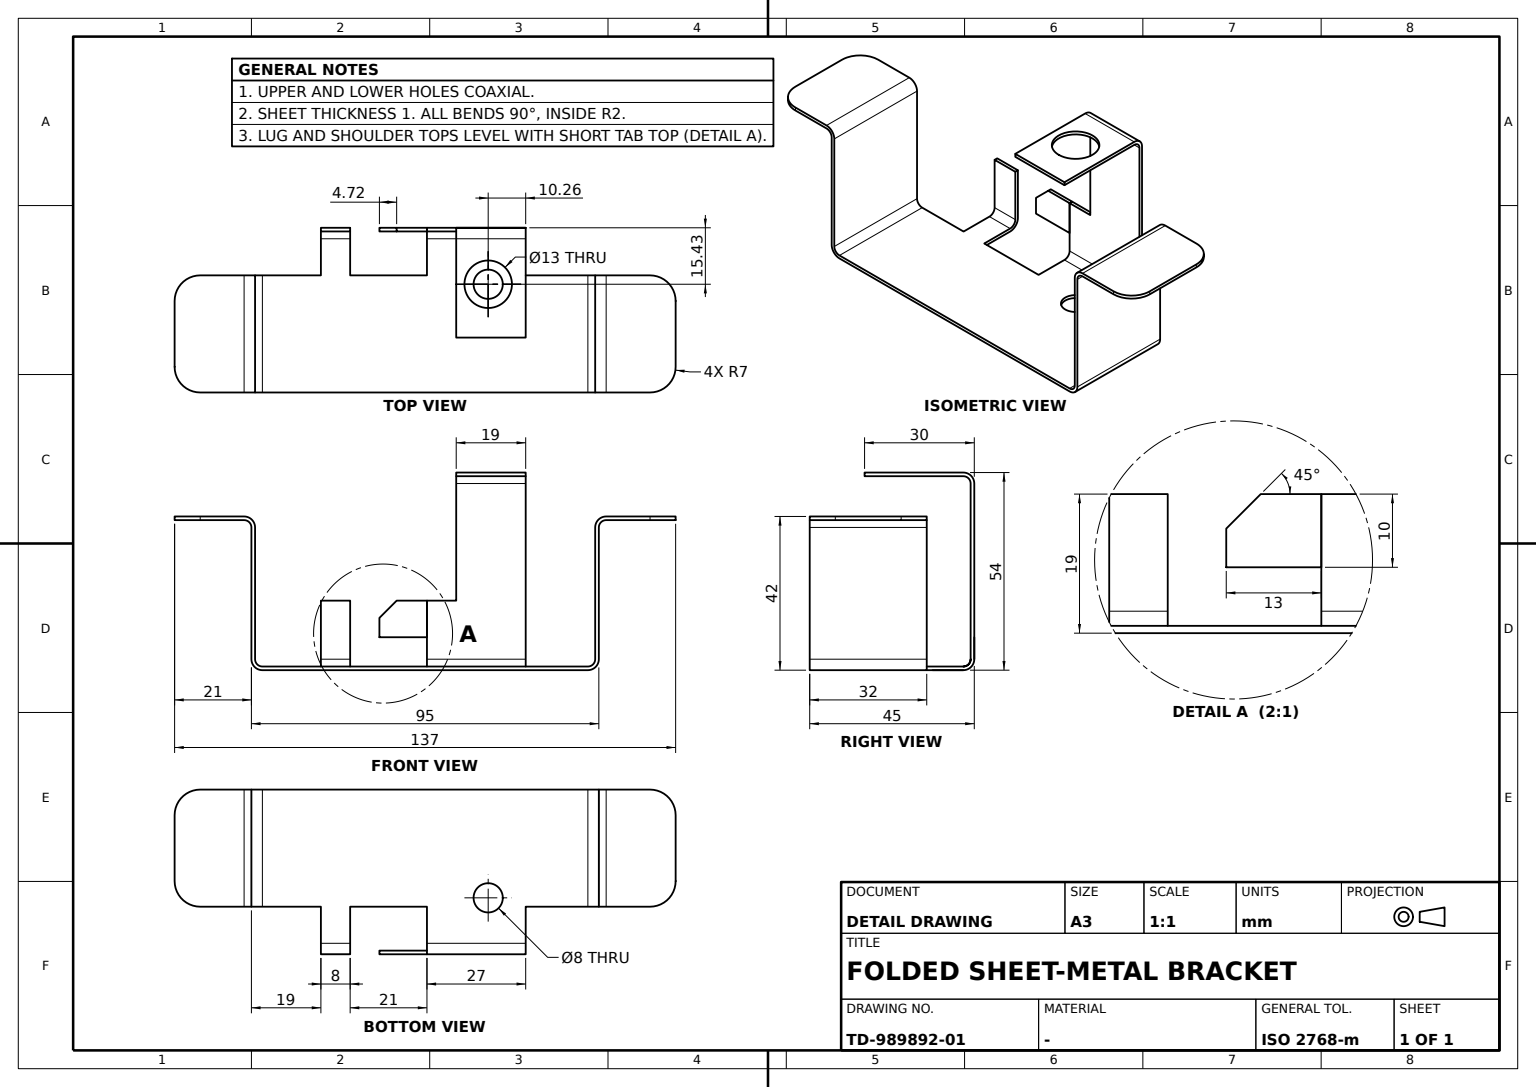
solid
v1 (27.5,26,53)
v2 (8.5,26,53)
e1 v1 v2 LINE
v3 (27.5,29,50)
e2 v3 v1 CIRCLE(AX(P(27.5,26,50),D(1,0,0),D(0,0,-1)),3)
v4 (8.5,29,50)
e3 v3 v4 LINE
e4 v4 v2 CIRCLE(AX(P(8.5,26,50),D(1,0,0),D(0,0,-1)),3)
face CYL(AX(P(18,26,50),D(-1,0,0),D(0,1,0)),3) [-e1 -e2 e3 e4]
v5 (-61.5,16,41)
v6 (-49.5,16,41)
e5 v5 v6 LINE
v7 (-68.5,9,41)
e6 v5 v7 CIRCLE(AX(P(-61.5,9,41),D(0,0,1),D(1,0,0)),7)
v8 (-68.5,-9,41)
e7 v8 v7 LINE
v9 (-61.5,-16,41)
e8 v8 v9 CIRCLE(AX(P(-61.5,-9,41),D(0,0,1),D(1,0,0)),7)
v10 (-49.5,-16,41)
e9 v10 v9 LINE
e10 v10 v6 LINE
face PLANE(AX(P(-47.5,0,41),D(0,0,1),D(0,1,0))) [-e5 e6 -e7 e8 -e9 e10]
v11 (-46.5,16,2)
v12 (-44.5,16,0)
e11 v11 v12 CIRCLE(AX(P(-44.5,16,2),D(0,-1,0),D(0,0,-1)),2)
v13 (-28.5,16,0)
e12 v12 v13 LINE
v14 (-28.5,16,-1)
e13 v13 v14 LINE
v15 (-44.5,16,-1)
e14 v15 v14 LINE
v16 (-47.5,16,2)
e15 v16 v15 CIRCLE(AX(P(-44.5,16,2),D(0,-1,0),D(0,0,-1)),3)
v17 (-47.5,16,38)
e16 v17 v16 LINE
v18 (-49.5,16,40)
e17 v18 v17 CIRCLE(AX(P(-49.5,16,38),D(0,-1,0),D(0,0,-1)),2) rev
v19 (-61.5,16,40)
e18 v18 v19 LINE
e19 v5 v19 LINE
v20 (-46.5,16,38)
e20 v6 v20 CIRCLE(AX(P(-49.5,16,38),D(0,-1,0),D(0,0,-1)),3) rev
e21 v11 v20 LINE
face PLANE(AX(P(47.5,16,0),D(0,-1,0),D(-1,0,0))) rev [e11 e12 e13 -e14 -e15 -e16 -e17 e18 -e19 e5 e20 -e21]
v21 (49.5,16,40)
v22 (49.5,-16,40)
e22 v21 v22 LINE
v23 (61.5,16,40)
e23 v21 v23 LINE
v24 (68.5,9,40)
e24 v24 v23 CIRCLE(AX(P(61.5,9,40),D(0,0,1),D(1,0,0)),7)
v25 (68.5,-9,40)
e25 v25 v24 LINE
v26 (61.5,-16,40)
e26 v26 v25 CIRCLE(AX(P(61.5,-9,40),D(0,0,1),D(1,0,0)),7)
e27 v26 v22 LINE
face PLANE(AX(P(-47.5,0,40),D(0,0,1),D(0,1,0))) rev [-e22 e23 -e24 -e25 -e26 e27]
v27 (-47.5,-16,2)
e28 v16 v27 LINE
v28 (-44.5,-16,-1)
e29 v15 v28 LINE
e30 v27 v28 CIRCLE(AX(P(-44.5,-16,2),D(0,1,0),D(0,0,1)),3) rev
face CYL(AX(P(-44.5,0,2),D(0,-1,0),D(0,0,-1)),3) [-e28 e15 e29 -e30]
v29 (-44.5,-16,0)
e31 v12 v29 LINE
v30 (-46.5,-16,2)
e32 v11 v30 LINE
e33 v30 v29 CIRCLE(AX(P(-44.5,-16,2),D(0,1,0),D(0,0,1)),2) rev
face CYL(AX(P(-44.5,0,2),D(0,-1,0),D(0,0,-1)),2) rev [-e31 -e11 e32 e33]
v31 (0.5,26,-1)
v32 (0.5,29,2)
e34 v31 v32 CIRCLE(AX(P(0.5,26,2),D(1,0,0),D(0,0,-1)),3)
v33 (27.5,29,2)
e35 v33 v32 LINE
v34 (27.5,26,-1)
e36 v34 v33 CIRCLE(AX(P(27.5,26,2),D(1,0,0),D(0,0,-1)),3)
e37 v34 v31 LINE
face CYL(AX(P(14,26,2),D(-1,0,0),D(0,0,-1)),3) [e34 -e35 -e36 e37]
v35 (17.243708,7.074732,52)
e38 v35 v35 CIRCLE(AX(P(17.243708,13.574732,52),D(0,0,1),D(0,-1,0)),6.5)
v36 (8.5,-1,52)
v37 (27.5,-1,52)
e39 v36 v37 LINE
v38 (8.5,26,52)
e40 v38 v36 LINE
v39 (27.5,26,52)
e41 v39 v38 LINE
e42 v37 v39 LINE
face PLANE(AX(P(18,28,52),D(0,0,1),D(-1,0,0))) rev [e38] [-e39 -e40 -e41 -e42]
v40 (0.5,16,-1)
e43 v40 v31 LINE
v41 (0.5,16,0)
e44 v41 v40 LINE
v42 (0.5,26,0)
e45 v41 v42 LINE
v43 (0.5,28,2)
e46 v42 v43 CIRCLE(AX(P(0.5,26,2),D(1,0,0),D(0,0,-1)),2)
v44 (0.5,28,18)
e47 v43 v44 LINE
v45 (0.5,29,18)
e48 v44 v45 LINE
e49 v45 v32 LINE
face PLANE(AX(P(0.5,29,21.5),D(1,0,0),D(0,0,-1))) rev [-e43 -e44 e45 e46 e47 e48 e49 -e34]
v46 (-68.5,-9,40)
e50 v8 v46 LINE
v47 (-68.5,9,40)
e51 v7 v47 LINE
e52 v47 v46 LINE
face PLANE(AX(P(-68.5,0,41),D(1,0,0),D(0,1,0))) rev [-e50 e7 e51 e52]
v48 (47.5,-16,38)
e53 v22 v48 CIRCLE(AX(P(49.5,-16,38),D(0,1,0),D(0,0,1)),2) rev
v49 (47.5,16,38)
e54 v49 v48 LINE
e55 v21 v49 CIRCLE(AX(P(49.5,16,38),D(0,-1,0),D(0,0,-1)),2)
face CYL(AX(P(49.5,0,38),D(0,-1,0),D(-1,0,0)),2) rev [e22 e53 -e54 -e55]
v50 (-28.5,26,0)
v51 (-20.5,26,0)
e56 v50 v51 LINE
e57 v13 v50 LINE
v52 (44.5,-16,0)
e58 v52 v29 LINE
v53 (44.5,16,0)
e59 v52 v53 LINE
v54 (27.5,16,0)
e60 v54 v53 LINE
v55 (27.5,26,0)
e61 v54 v55 LINE
e62 v55 v42 LINE
v56 (-20.5,16,0)
e63 v56 v41 LINE
e64 v56 v51 LINE
v57 (21.243708,13.574732,0)
e65 v57 v57 CIRCLE(AX(P(17.243708,13.574732,0),D(0,0,1),D(1,0,0)),4)
face PLANE(AX(P(0.5,16,0),D(0,0,1),D(1,0,0))) [-e56 -e57 -e12 e31 -e58 e59 -e60 e61 e62 -e45 -e63 e64] [-e65]
v58 (-28.5,29,18)
v59 (-20.5,29,18)
e66 v58 v59 LINE
v60 (-28.5,28,18)
e67 v60 v58 LINE
v61 (-20.5,28,18)
e68 v60 v61 LINE
e69 v61 v59 LINE
face PLANE(AX(P(4.5,29,18),D(0,0,-1),D(1,0,0))) rev [-e66 -e67 e68 e69]
v62 (27.5,-1,53)
e70 v62 v1 LINE
e71 v37 v62 LINE
v63 (27.5,28,50)
e72 v63 v39 CIRCLE(AX(P(27.5,26,50),D(1,0,0),D(0,0,-1)),2)
v64 (27.5,28,2)
e73 v64 v63 LINE
e74 v55 v64 CIRCLE(AX(P(27.5,26,2),D(1,0,0),D(0,0,-1)),2)
v65 (27.5,16,-1)
e75 v54 v65 LINE
e76 v65 v34 LINE
e77 v33 v3 LINE
face PLANE(AX(P(27.5,12.5,53),D(1,0,0),D(0,1,0))) [-e70 -e71 e42 -e72 -e73 -e74 -e61 e75 e76 e36 e77 e2]
v66 (-46.5,-16,38)
e78 v10 v66 CIRCLE(AX(P(-49.5,-16,38),D(0,1,0),D(0,0,1)),3)
e79 v66 v20 LINE
face CYL(AX(P(-49.5,0,38),D(0,1,0),D(1,0,0)),3) [-e20 -e10 e78 e79]
v67 (61.5,-16,41)
v68 (68.5,-9,41)
e80 v67 v68 CIRCLE(AX(P(61.5,-9,41),D(0,0,1),D(1,0,0)),7)
e81 v67 v26 LINE
e82 v68 v25 LINE
face CYL(AX(P(61.5,-9,41),D(0,0,1),D(0,-1,0)),7) [-e80 e81 e26 -e82]
v69 (49.5,16,41)
v70 (49.5,-16,41)
e83 v69 v70 LINE
e84 v67 v70 LINE
v71 (68.5,9,41)
e85 v71 v68 LINE
v72 (61.5,16,41)
e86 v71 v72 CIRCLE(AX(P(61.5,9,41),D(0,0,1),D(1,0,0)),7)
e87 v72 v69 LINE
face PLANE(AX(P(-47.5,0,41),D(0,0,1),D(0,1,0))) [e83 -e84 e80 -e85 e86 e87]
e88 v19 v47 CIRCLE(AX(P(-61.5,9,40),D(0,0,1),D(1,0,0)),7)
face CYL(AX(P(-61.5,9,41),D(0,0,1),D(0,1,0)),7) [-e6 e19 e88 -e51]
e89 v30 v66 LINE
face PLANE(AX(P(-46.5,0,0),D(-1,0,0),D(0,-1,0))) rev [e21 -e79 -e89 -e32]
v73 (-20.5,28,2)
e90 v61 v73 LINE
e91 v51 v73 CIRCLE(AX(P(-20.5,26,2),D(-1,0,0),D(0,0,1)),2) rev
v74 (-20.5,16,-1)
e92 v56 v74 LINE
v75 (-20.5,26,-1)
e93 v74 v75 LINE
v76 (-20.5,29,2)
e94 v75 v76 CIRCLE(AX(P(-20.5,26,2),D(-1,0,0),D(0,0,1)),3) rev
e95 v59 v76 LINE
face PLANE(AX(P(-20.5,21,-1),D(-1,0,0),D(0,1,0))) rev [-e69 e90 -e91 -e64 e92 e93 e94 -e95]
v77 (17.243708,7.074732,53)
e96 v77 v77 CIRCLE(AX(P(17.243708,13.574732,53),D(0,0,1),D(0,-1,0)),6.5)
face CYL(AX(P(17.243708,13.574732,52.5),D(0,0,1),D(1,0,0)),6.5) rev [-e38] [e96]
v78 (-28.5,26,-1)
v79 (-28.5,29,2)
e97 v78 v79 CIRCLE(AX(P(-28.5,26,2),D(-1,0,0),D(0,0,1)),3) rev
e98 v14 v78 LINE
v80 (-28.5,28,2)
e99 v50 v80 CIRCLE(AX(P(-28.5,26,2),D(-1,0,0),D(0,0,1)),2) rev
e100 v80 v60 LINE
e101 v79 v58 LINE
face PLANE(AX(P(-28.5,21,-1),D(-1,0,0),D(0,1,0))) [-e97 -e98 -e13 e57 e99 e100 e67 -e101]
e102 v80 v73 LINE
face PLANE(AX(P(8.5,28,41),D(0,-1,0),D(1,0,0))) [-e90 -e68 -e100 e102]
v81 (8.5,28,18)
e103 v81 v44 LINE
v82 (8.5,29,18)
e104 v81 v82 LINE
e105 v82 v45 LINE
face PLANE(AX(P(4.5,29,18),D(0,0,-1),D(1,0,0))) rev [-e48 -e103 e104 e105]
v83 (44.5,-16,-1)
v84 (44.5,16,-1)
e106 v83 v84 LINE
v85 (47.5,16,2)
e107 v85 v84 CIRCLE(AX(P(44.5,16,2),D(0,-1,0),D(0,0,-1)),3) rev
v86 (47.5,-16,2)
e108 v86 v85 LINE
e109 v86 v83 CIRCLE(AX(P(44.5,-16,2),D(0,1,0),D(0,0,1)),3)
face CYL(AX(P(44.5,0,2),D(0,1,0),D(0,0,-1)),3) [e106 -e107 -e108 e109]
v87 (8.5,-1,53)
e110 v2 v87 LINE
e111 v87 v62 LINE
face PLANE(AX(P(18,28,53),D(0,0,1),D(-1,0,0))) [e1 e110 e111 e70] [-e96]
e112 v82 v4 LINE
face PLANE(AX(P(8.5,29,41),D(0,-1,0),D(1,0,0))) rev [-e105 e112 -e3 -e77 e35 -e49]
v88 (8.5,28,50)
e113 v88 v38 CIRCLE(AX(P(8.5,26,50),D(1,0,0),D(0,0,-1)),2)
e114 v63 v88 LINE
face CYL(AX(P(18,26,50),D(-1,0,0),D(0,1,0)),2) rev [e72 e41 -e113 -e114]
v89 (46.5,-16,38)
e115 v70 v89 CIRCLE(AX(P(49.5,-16,38),D(0,1,0),D(0,0,1)),3) rev
v90 (46.5,-16,2)
e116 v90 v89 LINE
e117 v90 v52 CIRCLE(AX(P(44.5,-16,2),D(0,1,0),D(0,0,1)),2)
v91 (-61.5,-16,40)
e118 v9 v91 LINE
v92 (-49.5,-16,40)
e119 v92 v91 LINE
v93 (-47.5,-16,38)
e120 v92 v93 CIRCLE(AX(P(-49.5,-16,38),D(0,1,0),D(0,0,1)),2)
e121 v93 v27 LINE
e122 v83 v28 LINE
e123 v48 v86 LINE
face PLANE(AX(P(-47.5,-16,0),D(0,1,0),D(1,0,0))) rev [-e81 e84 e115 -e116 e117 e58 -e33 e89 -e78 e9 e118 -e119 e120 e121 e30 -e122 -e109 -e123 -e53 -e27]
e124 v46 v91 CIRCLE(AX(P(-61.5,-9,40),D(0,0,1),D(1,0,0)),7)
face CYL(AX(P(-61.5,-9,41),D(0,0,1),D(0,1,0)),7) [-e8 e50 e124 -e118]
v94 (46.5,16,38)
e125 v94 v89 LINE
v95 (46.5,16,2)
e126 v95 v94 LINE
e127 v90 v95 LINE
face PLANE(AX(P(46.5,0,0),D(1,0,0),D(0,1,0))) rev [-e125 -e126 -e127 e116]
e128 v95 v53 CIRCLE(AX(P(44.5,16,2),D(0,-1,0),D(0,0,-1)),2) rev
face CYL(AX(P(44.5,0,2),D(0,1,0),D(0,0,-1)),2) rev [e128 -e59 -e117 e127]
e129 v64 v43 LINE
face CYL(AX(P(14,26,2),D(-1,0,0),D(0,0,-1)),2) rev [-e46 -e62 e74 e129]
e130 v71 v24 LINE
e131 v72 v23 LINE
face CYL(AX(P(61.5,9,41),D(0,0,1),D(0,-1,0)),7) [-e86 e130 e24 -e131]
e132 v65 v84 LINE
e133 v78 v75 LINE
e134 v74 v40 LINE
v96 (21.243708,13.574732,-1)
e135 v96 v96 CIRCLE(AX(P(17.243708,13.574732,-1),D(0,0,1),D(1,0,0)),4)
face PLANE(AX(P(0.5,16,-1),D(0,0,1),D(1,0,0))) rev [e43 -e37 -e76 e132 -e106 e122 -e29 e14 e98 e133 -e93 e134] [e135]
e136 v93 v17 LINE
e137 v92 v18 LINE
face CYL(AX(P(-49.5,0,38),D(0,1,0),D(1,0,0)),2) rev [-e136 -e120 e137 e17]
face PLANE(AX(P(-47.5,0,0),D(-1,0,0),D(0,-1,0))) [e136 e16 e28 -e121]
e138 v79 v76 LINE
face PLANE(AX(P(8.5,29,41),D(0,-1,0),D(1,0,0))) rev [e66 e95 -e138 e101]
e139 v36 v87 LINE
e140 v81 v88 LINE
face PLANE(AX(P(8.5,12.5,53),D(1,0,0),D(0,1,0))) rev [e40 e139 -e110 -e4 -e112 -e104 e140 e113]
face CYL(AX(P(17.243708,13.574732,-0.5),D(0,0,1),D(1,0,0)),4) rev [e65] [-e135]
face PLANE(AX(P(-47.5,0,40),D(0,0,1),D(0,1,0))) rev [-e124 -e52 -e88 -e18 -e137 e119]
face PLANE(AX(P(8.5,28,41),D(0,-1,0),D(1,0,0))) [-e140 e103 -e47 -e129 e73 e114]
e141 v69 v94 CIRCLE(AX(P(49.5,16,38),D(0,-1,0),D(0,0,-1)),3)
face CYL(AX(P(49.5,0,38),D(0,-1,0),D(-1,0,0)),3) [e141 e125 -e115 -e83]
e142 v49 v85 LINE
face PLANE(AX(P(47.5,16,0),D(0,-1,0),D(-1,0,0))) rev [-e132 -e75 e60 -e128 e126 -e141 -e87 e131 -e23 e55 e142 e107]
face CYL(AX(P(14,26,2),D(-1,0,0),D(0,0,-1)),2) rev [e56 e91 -e102 -e99]
face PLANE(AX(P(47.5,16,0),D(0,-1,0),D(-1,0,0))) rev [-e92 e63 e44 -e134]
face CYL(AX(P(14,26,2),D(-1,0,0),D(0,0,-1)),3) [-e133 e97 e138 -e94]
face PLANE(AX(P(18,-1,53),D(0,1,0),D(1,0,0))) rev [e39 e71 -e111 -e139]
face PLANE(AX(P(68.5,0,41),D(-1,0,0),D(0,1,0))) rev [e25 -e130 e85 e82]
face PLANE(AX(P(47.5,0,0),D(1,0,0),D(0,1,0))) [e54 e123 e108 -e142]
solid
v97 (-12.5,29,8)
v98 (-12.5,29,13.283)
e143 v97 v98 LINE
v99 (-7.783,29,18)
e144 v99 v98 LINE
v100 (0.5,29,18)
e145 v100 v99 LINE
v101 (0.5,29,8)
e146 v100 v101 LINE
e147 v97 v101 LINE
face PLANE(AX(P(0,29,0),D(0,1,0),D(-1,0,0))) [e143 -e144 -e145 e146 -e147]
v102 (-7.783,28,18)
e148 v102 v99 LINE
v103 (0.5,28,18)
e149 v103 v102 LINE
e150 v103 v100 LINE
face PLANE(AX(P(-7.783,29,18),D(0,0,-1),D(1,0,0))) rev [-e148 -e149 e150 e145]
v104 (-12.5,28,13.283)
e151 v104 v98 LINE
v105 (-12.5,28,8)
e152 v105 v97 LINE
e153 v105 v104 LINE
face PLANE(AX(P(-12.5,29,8),D(1,0,0),D(0,0,1))) rev [e151 -e143 -e152 e153]
e154 v102 v104 LINE
v106 (0.5,28,8)
e155 v105 v106 LINE
e156 v103 v106 LINE
face PLANE(AX(P(0,28,0),D(0,1,0),D(-1,0,0))) rev [e154 -e153 e155 -e156 e149]
face PLANE(AX(P(-12.5,29,13.283),D(0.707106781,0,-0.707106781),D(0.707106781,0,0.707106781))) rev [e148 e144 -e151 -e154]
e157 v106 v101 LINE
face PLANE(AX(P(0.5,29,18),D(-1,0,0),D(0,0,-1))) rev [-e146 -e150 e156 e157]
face PLANE(AX(P(0.5,29,8),D(0,0,1),D(-1,0,0))) rev [-e157 -e155 e152 e147]
